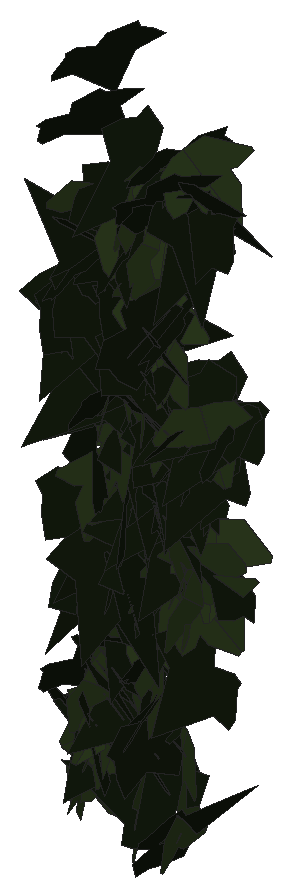
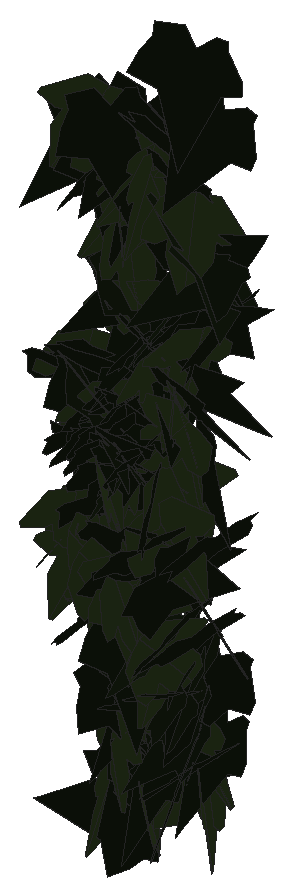
# SketchUp Ruby script. Lengths in inches.
U = 1.inch
M = Sketchup.active_model
def pt(a) = Geom::Point3d.new(a.map { |v| v * U })
def face(e, loops, mat)
  f = e.add_face(loops[0].map { |a| pt(a) })
  loops[1..].each { |l| e.add_face(l.map { |a| pt(a) }).erase! }
  f.material = f.back_material = mat if mat
  f
end
# faces: each face lists its corners as indices into pts; further lists are holes
def faces(e, pts, list, mat = nil) = list.each { |f| face(e, (f[0].is_a?(Array) ? f : [f]).map { |l| l.map { |i| pts[i] } }, mat) }
# xy, xz, yz: faces in a plane at the given z, y or x. An outline is a flat list of corners, or four numbers for a rectangle; further outlines are holes
def ring(l) = l.size == 4 ? [[l[0], l[1]], [l[2], l[1]], [l[2], l[3]], [l[0], l[3]]] : l.each_slice(2).to_a
def flat(e, list, mat, &to3) = list.each { |f| face(e, (f[0].is_a?(Array) ? f : [f]).map { |l| ring(l).map { |u, v| to3.(u, v) } }, mat) }
def xy(e, z, list, mat = nil) = flat(e, list, mat) { |x, y| [x, y, z] }
def xz(e, y, list, mat = nil) = flat(e, list, mat) { |x, z| [x, y, z] }
def yz(e, x, list, mat = nil) = flat(e, list, mat) { |y, z| [x, y, z] }
def lines(e, pts, list) = list.each { |a, b| e.add_line(pt(pts[a]), pt(pts[b])) }
# prism: a flat outline (further loops are holes) pulled along v
def prism(e, loops, v, mat = nil)
  f = face(e, loops, mat); d = Geom::Vector3d.new(v.map { |x| x * U })
  f.pushpull(f.normal.samedirection?(d) ? d.length : -d.length)
end
def box(e, o, s, mat = nil) = prism(e, [[o, [o[0] + s[0], o[1], o[2]], [o[0] + s[0], o[1] + s[1], o[2]], [o[0], o[1] + s[1], o[2]]]], [0, 0, s[2]], mat)
def at(x, y, z, deg = 0) = Geom::Transformation.translation(pt([x, y, z])) * Geom::Transformation.rotation(ORIGIN, Z_AXIS, deg.degrees)
def axes(o, x, y, z) = Geom::Transformation.new([*x, 0, *y, 0, *z, 0, *pt(o).to_a, 1])
def part(name) = M.definitions.add(name)
# library, detail: a bought-in or finely detailed component or shape, given as its bounding box
def library(name, o, s) = part(name).tap { |d| box(d.entities, o, s) }
def detail(e, o, s) = box(e.add_group.entities, o, s)
def put(e, d, t, mat = nil) = e.add_instance(d, t).tap { |i| i.material = mat if mat }
def group(e, t, mat = nil) = e.add_group.tap { |g| g.transformation = t; g.material = mat if mat }.entities
root = M.entities
M.materials.add("efeu1").color = [18, 25, 13]
M.materials.add("efeu2").color = [43, 57, 29]
c1 = part("ivyleaf_9")
p = [[1.54,2.16,1.25],[1.36,2.04,1.19],[-0.21,0.99,0.68],[-0.71,1.11,0.82],[-0.85,0.86,0.67],[-0.8,0.17,0.21],
  [-0.9,-0.01,0.1],[-0.67,-0.16,-0.02],[-0.08,-0.08,-0.05],[-0.03,-0.6,-0.4],[0.65,-0.88,-0.66],[0.83,-0.6,-0.49],
  [1.29,-0.42,-0.43],[1.8125,-0.07,-0.26],[1.21,0.44,0.15]]
faces(c1.entities,p,[[0,1,2,3,4,5,6,7,8,9,10,11,12,13,14]],"efeu1")
c2 = part("ivyleaf_10")
p = [[0,0.5,-0.03],[-0.0625,2.02,-0.43],[-0.19,2.01,-0.46],[-0.54,1.05,-0.29],[-0.52,0.625,-0.18],[-0.83,0.76,-0.28],
  [-1.16,0.64,-0.33],[-1.15,0.33,-0.24],[-0.77,-0.39,0.02],[-0.3,-0.51,0.16],[0.04,-0.48,0.23],[-0.02,2.01,-0.4375],
  [-0.06,2.01,-0.43],[0.04,-0.49,0.23],[0.67,-0.49,0.14],[1.38,0.36,-0.2],[1.375,0.51,-0.24],[0.81,0.65,-0.19],
  [0.62,0.59,-0.15],[0.6,1.09,-0.28],[0.5,1.23,-0.31]]
faces(c2.entities,p,[[0,1,2,3,4,5,6,7,8,9,10],[11,12,0,13,14,15,16,17,18,19,20]],"efeu2")
put(root,c1,axes([33.9,223.34,230.51],[0.00154,0.42012,0.27111],[-0.14788,0.25936,-0.40108],[-0.47763,-0.07894,0.12505]))
put(root,c1,axes([33.63,223.56,224.36],[0.44451,0.03173,-0.22672],[-0.22814,0.02019,-0.44446],[-0.01905,0.49858,0.03243]))
put(root,c1,axes([33.47,223.96,227.15],[0.1499,-0.43389,-0.19816],[0.01697,0.21244,-0.45231],[0.4767,0.12887,0.07842]))
put(root,c2,axes([33.78,223.74,223.54],[0.20397,-0.43865,-0.12641],[-0.02704,0.1266,-0.48295],[0.4557,0.20385,0.02792]))
put(root,c1,axes([34.06,223.51,228.01],[0.00848,0.06213,-0.49605],[-0.49993,0.00276,-0.0082],[0.00172,0.49612,0.06217]))
put(root,c1,axes([33.59,223.62,229.9],[0.20274,-0.41482,-0.19189],[-0.09111,0.16903,-0.46166],[0.44788,0.22216,-0.00705]))
put(root,c1,axes([34.1,223.64,230.47],[0.04588,0.02887,0.49705],[-0.45036,0.21524,0.02907],[-0.21229,-0.45038,0.04575]))
put(root,c1,axes([33.92,223.87,226.3125],[-0.45711,0.12817,-0.1569],[0.15505,-0.02792,-0.47453],[-0.1304,-0.48249,-0.01422]))
put(root,c1,axes([33.8,223.84,229.95],[-0.28838,-0.40509,0.05235],[-0.01287,-0.05504,-0.49679],[0.40825,-0.28788,0.02132]))
put(root,c1,axes([33.53,223.69,230.83],[0.49721,-0.02109,0.04834],[0.05123,0.08398,-0.49023],[0.01256,0.49245,0.08567]))
put(root,c2,axes([34.03,223.6,224.125],[0.27092,-0.16584,-0.38613],[-0.31496,0.22402,-0.3172],[0.27822,0.4151,0.01692]))
put(root,c1,axes([33.8125,223.4,232.65],[0.24869,0.41729,0.11842],[0.03901,0.11443,-0.48516],[-0.43201,0.25055,0.02436]))
put(root,c1,axes([33.62,224.1875,225.86],[0.03188,-0.49682,-0.04636],[0.06993,0.05044,-0.49251],[0.49406,0.02492,0.0727]))
put(root,c1,axes([33.77,224.01,224.02],[-0.07048,0.02019,0.4946],[-0.01004,-0.49954,0.01896],[0.49491,-0.00726,0.07082]))
put(root,c2,axes([33.95,223.78,231.38],[-0.43459,-0.24681,-0.01471],[0.00913,0.0137,-0.49973],[0.24708,-0.43462,-0.0074]))
put(root,c2,axes([34.14,224.14,227.16],[-0.33842,-0.21683,0.29742],[-0.25069,-0.16003,-0.40193],[0.26949,-0.42116,-0.00041]))
put(root,c1,axes([33.88,223.39,225.12],[0.24742,0.42796,0.07509],[0.03871,0.06436,-0.49433],[-0.43277,0.25042,-0.00128]))
put(root,c1,axes([33.86,224.26,223.84],[-0.22406,-0.37999,0.23538],[0.0143,-0.26925,-0.42107],[0.44676,-0.18196,0.13152]))
put(root,c1,axes([34,223.66,233.52],[0.14051,0.47873,-0.03276],[-0.01335,-0.03022,-0.49891],[-0.47967,0.14108,0.00429]))
put(root,c1,axes([34.15,223.78,229.05],[-0.47057,-0.1429,0.09024],[-0.08634,-0.02626,-0.49179],[0.14529,-0.47843,0.00004]))
put(root,c1,axes([33.9,223.83,224.04],[0.28906,-0.21291,-0.34801],[-0.29246,0.18922,-0.35869],[0.28444,0.41093,-0.01514]))
put(root,c1,axes([33.97,224.39,226.65],[0.01619,-0.04905,-0.49732],[0.16578,-0.46888,0.05164],[-0.47144,-0.16656,0.00108]))
put(root,c2,axes([33.87,223.76,229.64],[0.16446,0.46778,0.06428],[0.00821,0.06522,-0.49566],[-0.47211,0.16408,0.01377]))
put(root,c1,axes([33.76,223.94,224.53],[0.45939,-0.19291,-0.04182],[-0.03541,0.02368,-0.49818],[0.19419,0.46068,0.0081]))
put(root,c2,axes([34.125,223.84,227.65],[-0.23925,-0.39616,0.18926],[-0.04257,-0.19359,-0.45903],[0.43697,-0.23576,0.0589]))
put(root,c2,axes([34.0625,223.91,228.97],[0.28961,-0.40737,0.01319],[0.00784,-0.01061,-0.49983],[0.40751,0.28971,0.00024]))
put(root,c1,axes([34.32,223.91,229.02],[-0.49444,0.06662,0.03306],[-0.03522,-0.01397,-0.49856],[-0.0655,-0.49535,0.01851]))
put(root,c2,axes([34.14,224.25,225.5],[-0.15259,-0.31826,0.35415],[-0.02417,-0.36624,-0.33954],[0.47553,-0.12074,0.09638]))
put(root,c1,axes([33.85,223.74,230.09],[0.13066,-0.46006,-0.14586],[0.00748,0.15303,-0.47595],[0.48257,0.1222,0.04688]))
put(root,c2,axes([34.22,223.8,224.625],[0.23833,0.32811,-0.29248],[-0.16769,-0.23967,-0.40551],[-0.4063,0.29138,-0.0042]))
put(root,c1,axes([33.875,223.72,225.02],[0.38873,-0.31106,0.04615],[0.03455,-0.03068,-0.49786],[0.31256,0.39025,-0.00236]))
put(root,c1,axes([34.14,223.87,226.48],[-0.1966,-0.45859,0.03224],[-0.008,-0.03165,-0.49893],[0.45965,-0.1967,0.00511]))
put(root,c2,axes([34.11,223.46,224.86],[-0.13206,-0.28655,-0.38788],[0.18444,0.34157,-0.31514],[0.44558,-0.22632,0.01549]))
put(root,c1,axes([34.05,224.25,225.61],[-0.0125,-0.46121,0.19268],[-0.00571,-0.1926,-0.46138],[0.49981,-0.01374,-0.00045]))
put(root,c1,axes([33.92,223.9,224.83],[0.43049,-0.2535,0.02037],[0.01944,-0.00713,-0.49957],[0.25357,0.43092,0.00372]))
put(root,c1,axes([34.49,223.55,231.1],[-0.38201,0.322,0.01959],[-0.01337,0.01454,-0.49961],[-0.32232,-0.38224,-0.00249]))
put(root,c2,axes([34.06,223.61,223.56],[-0.40057,-0.08418,-0.28715],[0.28601,0.03336,-0.40876],[0.08798,-0.49173,0.02143]))
put(root,c2,axes([33.96,223.97,228.49],[0.36637,0.05604,0.33561],[0.32079,0.10751,-0.36815],[-0.11343,0.48508,0.04282]))
put(root,c2,axes([34.25,223.91,225.4],[-0.142,-0.43792,-0.19509],[0.1003,0.17183,-0.45871],[0.4688,-0.16941,0.03904]))
put(root,c2,axes([34.39,223.5625,228.23],[0.38045,-0.25851,-0.19604],[-0.15461,0.12115,-0.4598],[0.28522,0.41048,0.01225]))
put(root,c1,axes([34.25,223.93,223.9375],[0.42717,-0.02527,-0.25863],[-0.25766,0.0234,-0.42786],[0.03373,0.49881,0.00697]))
put(root,c2,axes([34.3,223.81,228.95],[-0.3657,0.32259,-0.11044],[0.01974,-0.14165,-0.47911],[-0.3404,-0.35478,0.09087]))
put(root,c1,axes([34.03,223.95,224.9375],[0.41077,-0.28321,0.03252],[0.03359,-0.00855,-0.4988],[0.28309,0.41197,0.012]))
put(root,c1,axes([34.46,223.31,229.12],[0.03499,0.49695,0.04258],[0.0167,0.04149,-0.498],[-0.49849,0.03627,-0.01369]))
put(root,c1,axes([34.27,224.32,226.89],[-0.13061,-0.48213,-0.02217],[0.05937,0.00674,-0.49642],[0.47898,-0.1323,0.05548]))
put(root,c1,axes([34.52,224.1875,224.65],[-0.40088,-0.24617,0.1694],[-0.04382,-0.23195,-0.44077],[0.29559,-0.36824,0.16439]))
put(root,c2,axes([34.375,223.93,229.33],[0.01008,0.47814,-0.14586],[0.00284,-0.14595,-0.47822],[-0.49989,0.00881,-0.00566]))
put(root,c1,axes([34.26,224.15,227.47],[0.04534,-0.07717,-0.49192],[0.41319,-0.26983,0.08041],[-0.27788,-0.41381,0.03931]))
put(root,c1,axes([34.23,223.89,229.93],[0.25344,-0.43101,-0.00107],[0.00982,0.00701,-0.49985],[0.4309,0.25335,0.01202]))
put(root,c1,axes([34.35,223.65,231.72],[-0.30287,-0.17579,-0.35688],[0.33179,0.13586,-0.34851],[0.2195,-0.44793,0.03436]))
put(root,c2,axes([34.41,224.07,223.37],[0.25899,-0.38727,0.18151],[0.13884,-0.12458,-0.4639],[0.40453,0.2907,0.04301]))
put(root,c2,axes([34.68,223.56,228.86],[0.25269,-0.21336,-0.375],[-0.18673,0.33769,-0.31796],[0.38894,0.30074,0.09098]))
put(root,c1,axes([34.78,223.73,232.26],[-0.49954,0.00885,-0.01952],[0.01949,-0.00203,-0.49962],[-0.00893,-0.49992,0.00169]))
put(root,c2,axes([34.66,223.97,226.0625],[-0.36834,-0.33801,0.00872],[-0.00623,-0.00611,-0.49992],[0.33807,-0.36839,0.00029]))
put(root,c1,axes([34.24,224.18,225.44],[0.26974,-0.40775,0.10478],[0.15551,-0.01914,-0.47482],[0.39122,0.28875,0.11649]))
put(root,c1,axes([34.97,223.84,223.25],[-0.16346,0.04365,0.47051],[-0.46675,0.06268,-0.16797],[-0.07365,-0.49413,0.02025]))
put(root,c2,axes([34.59,223.74,231.64],[0.01708,-0.40797,-0.28856],[0.06796,0.28794,-0.40307],[0.49506,-0.02545,0.06529]))
put(root,c1,axes([34.85,223.9,229.59],[-0.48516,0.11557,-0.03553],[0.0315,-0.02104,-0.49856],[-0.11673,-0.48601,0.01314]))
put(root,c1,axes([34.78,223.87,225.35],[-0.01221,0.49972,-0.01154],[0.00022,-0.01154,-0.49987],[-0.49985,-0.01221,0.00006]))
put(root,c1,axes([34.4,223.68,228.69],[0.49476,-0.07181,-0.00768],[-0.00762,0.00096,-0.49994],[0.07182,0.49482,-0.00014]))
put(root,c1,axes([34.41,223.61,226.42],[-0.18053,-0.07374,-0.4604],[0.43505,0.15098,-0.19477],[0.16775,-0.47092,0.00964]))
put(root,c2,axes([34.71,224.1875,226.13],[0.0259,-0.49102,0.09073],[0.00087,-0.09081,-0.49168],[0.49933,0.02563,-0.00385]))
put(root,c1,axes([34.51,224.07,228.01],[0.00314,-0.49545,0.06723],[0.01248,-0.06713,-0.49532],[0.49983,0.00479,0.01194]))
put(root,c1,axes([34.66,224.25,226.93],[-0.37567,-0.28602,-0.16451],[0.17761,0.0348,-0.46609],[0.27807,-0.40864,0.07545]))
put(root,c2,axes([34.57,223.5,231.32],[0.17734,0.35727,0.3015],[0.10046,0.28581,-0.39777],[-0.45657,0.20166,0.02959]))
put(root,c1,axes([34.52,223.75,229.53],[0.15371,-0.44957,-0.15577],[-0.01279,0.15973,-0.47363],[0.47561,0.14959,0.0376]))
put(root,c2,axes([34.86,223.62,225.1],[0.3242,-0.29626,-0.23901],[-0.16727,0.17113,-0.43902],[0.34193,0.36461,0.01185]))
put(root,c1,axes([34.65,224.18,226.42],[-0.1554,-0.46954,-0.07337],[0.03778,0.06474,-0.49435],[0.47373,-0.15918,0.01536]))
put(root,c2,axes([34.73,223.84,230.03],[0.43416,0.24533,-0.0363],[-0.02753,-0.02506,-0.49861],[-0.24647,0.43496,-0.00825]))
put(root,c1,axes([35.01,223.25,224.73],[-0.08007,0.40846,0.27704],[-0.0477,0.27294,-0.41621],[-0.49124,-0.09308,-0.00474]))
put(root,c2,axes([34.73,223.51,231.59],[0.00161,-0.20367,-0.45664],[0.16673,0.43072,-0.19152],[0.47138,-0.15166,0.06931]))
put(root,c1,axes([35.05,223.72,230.23],[-0.2662,0.41259,-0.0944],[0.00957,-0.10562,-0.48862],[-0.42314,-0.26194,0.04834]))
put(root,c2,axes([34.87,223.8125,230.77],[-0.09388,-0.4911,-0.0034],[0.00692,0.00214,-0.49995],[0.49106,-0.09391,0.00639]))
put(root,c2,axes([34.84,224.12,226.35],[0.34398,0.33629,-0.13633],[-0.12199,-0.06975,-0.47985],[-0.34175,0.36338,0.03406]))
put(root,c1,axes([35.11,224.08,227.93],[-0.48092,-0.02685,0.13415],[-0.13174,-0.04135,-0.48056],[0.03691,-0.49756,0.0327]))
put(root,c1,axes([34.72,223.68,229.76],[0.46495,-0.04893,-0.17728],[-0.17586,0.02272,-0.4675],[0.05381,0.49708,0.00392]))
put(root,c1,axes([34.81,224.2,227.81],[-0.25486,-0.42497,-0.06664],[0.04398,0.05131,-0.49541],[0.42791,-0.25839,0.01123]))
put(root,c1,axes([35.02,223.86,224.74],[-0.0811,0.40427,-0.28282],[0.06554,-0.27525,-0.41224],[-0.48901,-0.10394,-0.00835]))
put(root,c1,axes([34.87,223.41,224.55],[0.06557,-0.14698,-0.47339],[-0.22799,0.41506,-0.16045],[0.44014,0.2369,-0.01259]))
put(root,c2,axes([34.97,223.71,229.57],[0.46343,-0.12311,-0.14168],[-0.12937,0.06395,-0.47872],[0.13599,0.48037,0.02742]))
put(root,c1,axes([35.13,223.75,227.86],[-0.44578,0.21018,-0.08429],[0.0798,-0.02837,-0.49278],[-0.21193,-0.45279,-0.00825]))
put(root,c1,axes([34.79,223.3,230.05],[0.05941,0.10629,-0.48495],[-0.06904,0.48543,0.09794],[0.49163,0.05532,0.07235]))
put(root,c1,axes([35.08,223.95,227.8],[-0.4571,-0.20133,0.02303],[-0.02213,-0.00689,-0.49946],[0.20143,-0.45762,-0.00261]))
put(root,c2,axes([34.98,224,224.0625],[0.42537,-0.21594,-0.14976],[-0.07469,0.17385,-0.46282],[0.25195,0.41611,0.11565]))
put(root,c2,axes([34.9375,224.21,227.72],[0.22722,-0.43718,0.0851],[0.05042,-0.06967,-0.49255],[0.44252,0.23242,0.01243]))
put(root,c2,axes([35.01,223.77,231.96],[-0.43994,-0.23515,-0.03399],[0.02909,0.01769,-0.49884],[0.23581,-0.4409,-0.00189]))
put(root,c2,axes([35.15,223.85,231.3],[-0.36864,0.27574,0.19512],[-0.23234,0.00266,-0.44273],[-0.2452,-0.41709,0.12617]))
put(root,c1,axes([35.25,223.68,230.18],[-0.34853,0.35383,-0.05773],[0.00378,-0.07689,-0.49404],[-0.35849,-0.34481,0.05092]))
put(root,c2,axes([34.8,223.91,225.74],[0.39961,0.18672,0.23548],[0.18612,0.15383,-0.43783],[-0.23595,0.43758,0.05344]))
put(root,c1,axes([34.9,224.17,228.36],[-0.08064,-0.49066,0.05245],[-0.00039,-0.05308,-0.49717],[0.49345,-0.08022,0.00817]))
put(root,c1,axes([34.76,224.05,227.7],[0.22315,-0.43491,0.10517],[0.04363,-0.09581,-0.48879],[0.44531,0.22733,-0.00481]))
put(root,c1,axes([34.92,224.21,228.15],[-0.09409,-0.48757,0.05853],[-0.00126,-0.05936,-0.49646],[0.49107,-0.09357,0.00994]))
put(root,c1,axes([35.16,223.8125,232.39],[0.02026,0.46546,-0.18149],[-0.00335,-0.18151,-0.46588],[-0.49958,0.0201,-0.00424]))
put(root,c1,axes([34.89,223.64,222.78],[-0.01082,0.42707,-0.25979],[-0.00281,0.2598,0.4272],[0.49987,0.01071,-0.00322]))
put(root,c1,axes([35.45,224.08,227.79],[-0.37368,0.14028,0.30113],[-0.31004,0.01549,-0.39196],[-0.1193,-0.47967,0.07541]))
put(root,c1,axes([35.17,224.03,228.53],[-0.47645,-0.11138,-0.10288],[0.10792,-0.01078,-0.4881],[0.10651,-0.48732,0.03432]))
put(root,c2,axes([35.11,224.23,226.35],[-0.06493,-0.37781,0.321],[0.03589,-0.32647,-0.377],[0.49446,-0.02592,0.06952]))
put(root,c2,axes([35.08,223.91,226.86],[0.3613,-0.34561,-0.00391],[-0.00142,0.00416,-0.49998],[0.34563,0.3613,0.00202]))
put(root,c2,axes([35.14,223.8,223.2],[0.0336,-0.31024,-0.39067],[-0.00333,0.3914,-0.31111],[0.49886,0.02351,0.02423]))
put(root,c2,axes([35,223.5,231.18],[-0.11071,-0.29008,-0.39191],[0.21398,0.33221,-0.30634],[0.43812,-0.23556,0.05058]))
put(root,c1,axes([35.19,223.5,231.76],[0.20992,0.43951,-0.11297],[-0.06374,-0.09468,-0.4868],[-0.4493,0.21878,0.01628]))
put(root,c2,axes([35.09,223.92,228.51],[0.14533,0.46253,0.12223],[-0.06222,0.14494,-0.47447],[-0.47435,0.1227,0.09969]))
put(root,c1,axes([35,223.89,228.51],[0.04782,-0.39419,-0.30385],[-0.05111,0.29975,-0.39691],[0.49508,0.06902,-0.01163]))
put(root,c1,axes([35.4,223.8,228.5625],[-0.20099,0.45091,0.07928],[-0.04265,0.06777,-0.49355],[-0.45583,-0.20516,0.01122]))
put(root,c2,axes([35.09,223.69,231.8],[0.43415,0.24616,-0.03027],[-0.02641,-0.01479,-0.49908],[-0.2466,0.43496,0.00016]))
put(root,c2,axes([35.17,223.48,227.37],[-0.41485,0.27803,-0.02449],[0.01915,-0.01543,-0.4994],[-0.27845,-0.41528,0.00216]))
put(root,c1,axes([35.03,224.21,228.27],[-0.00257,-0.49506,-0.07008],[-0.00557,0.07011,-0.49503],[0.49996,-0.00176,-0.00587]))
put(root,c1,axes([35.14,223.22,232.03],[0.27955,0.39756,0.11747],[0.05013,0.10823,-0.48557],[-0.41151,0.28326,0.02065]))
put(root,c1,axes([35.38,223.77,228.67],[-0.00653,0.49612,-0.06179],[-0.04024,-0.06212,-0.49449],[-0.49834,-0.00149,0.04074]))
put(root,c1,axes([35.24,224.1,227.1875],[-0.23932,-0.41608,0.14001],[-0.07516,-0.11827,-0.47996],[0.43252,-0.25077,-0.00594]))
put(root,c1,axes([35.33,224.2,228.17],[-0.20398,-0.43701,0.13198],[0.00029,-0.14468,-0.47861],[0.4565,-0.19518,0.05927]))
put(root,c1,axes([35.66,223.95,228.78],[-0.45113,0.2155,0.00659],[-0.00777,-0.00097,-0.49994],[-0.21546,-0.45118,0.00422]))
put(root,c2,axes([35.45,223.75,226.9],[-0.38204,-0.32125,-0.02907],[0.02005,0.02132,-0.49914],[0.32194,-0.38255,-0.00341]))
put(root,c1,axes([35.68,224.14,228.99],[-0.48337,-0.07711,0.10204],[-0.08471,-0.10585,-0.48127],[0.09582,-0.48255,0.08927]))
put(root,c2,axes([35.37,224.14,226.55],[0.11811,-0.36058,0.32563],[0.13956,-0.29581,-0.37818],[0.46538,0.18022,0.03077]))
put(root,c2,axes([35.5,223.54,226.46],[-0.04175,-0.32831,-0.37479],[0.05308,0.37103,-0.33093],[0.49542,-0.06742,0.00388]))
put(root,c1,axes([35.3125,223.85,231.61],[0.0784,-0.49067,0.05567],[0.00904,-0.05493,-0.49689],[0.49373,0.07892,0.00026]))
put(root,c1,axes([35.59,224.36,226.5],[0.12733,-0.47872,-0.06796],[0.01227,-0.06706,0.49533],[-0.48336,-0.12781,-0.00533]))
put(root,c2,axes([35.5,224.06,227.04],[0.29334,0.40132,-0.05379],[-0.0469,-0.03231,-0.49675],[-0.40218,0.29648,0.01869]))
put(root,c1,axes([35.52,223.94,225.33],[-0.18053,-0.35021,0.30784],[-0.03886,-0.31766,-0.38417],[0.46465,-0.16263,0.08748]))
put(root,c1,axes([35.65,223.72,231.7],[-0.46963,-0.06536,-0.15866],[0.15695,0.02324,-0.47416],[0.06936,-0.49516,-0.00131]))
put(root,c2,axes([35.52,223.76,226.3],[0.20403,0.34964,0.29347],[-0.00731,0.32391,-0.38083],[-0.45642,0.15111,0.13729]))
put(root,c1,axes([35.72,224.1,228.96],[-0.42749,-0.25932,-0.00313],[0.00305,0.00101,-0.49999],[0.25932,-0.4275,0.00072]))
put(root,c1,axes([35.42,223.58,232.03],[0.4945,0.07397,-0.00129],[-0.00895,0.0512,-0.49729],[-0.07344,0.49184,0.05196]))
put(root,c2,axes([35.47,223.68,232.37],[0.2489,0.32716,0.28464],[0.10329,0.27402,-0.40527],[-0.42117,0.26054,0.06882]))
put(root,c2,axes([35.62,223.71,228.9],[-0.38469,-0.30197,-0.10405],[0.11297,0.02372,-0.48649],[0.29874,-0.39781,0.04998]))
